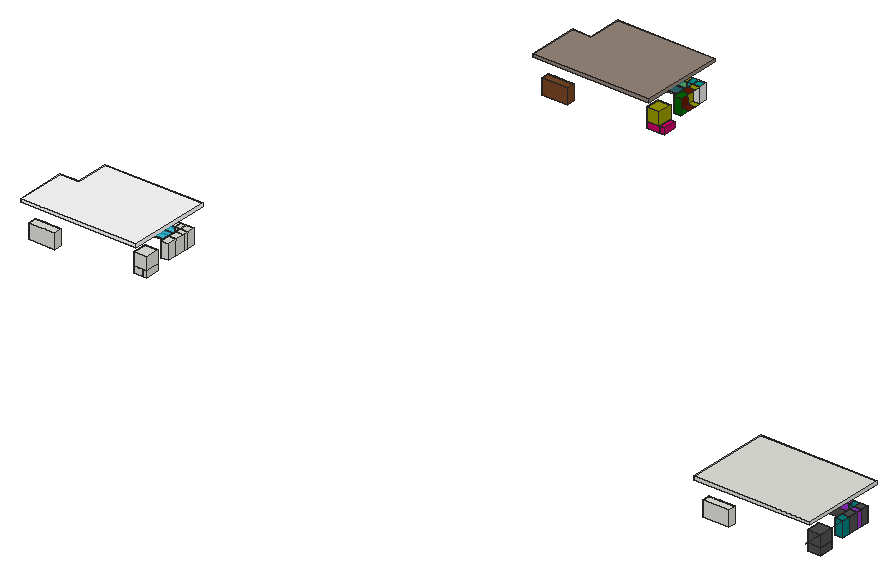
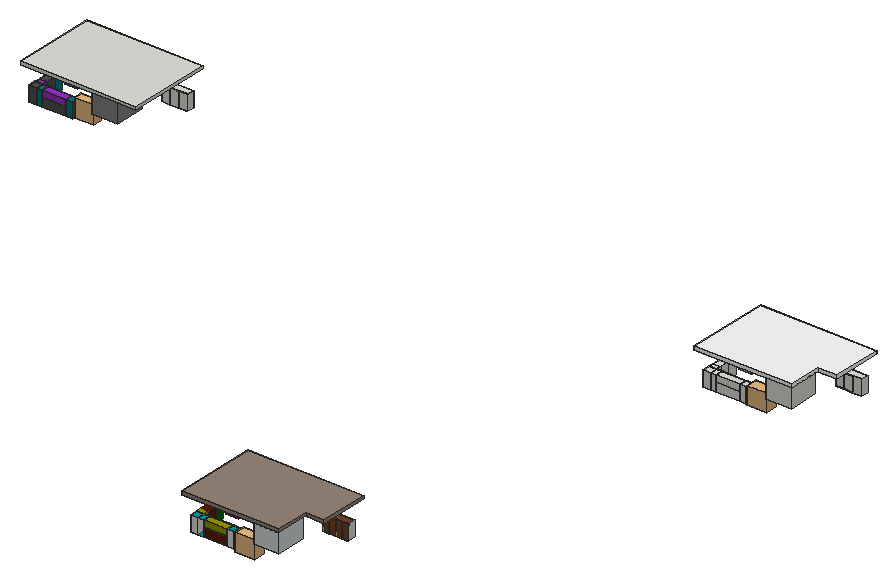
# SketchUp Ruby script. Lengths in inches.
U = 1.inch
M = Sketchup.active_model
def pt(a) = Geom::Point3d.new(a.map { |v| v * U })
def face(e, loops, mat)
  f = e.add_face(loops[0].map { |a| pt(a) })
  loops[1..].each { |l| e.add_face(l.map { |a| pt(a) }).erase! }
  f.material = f.back_material = mat if mat
  f
end
# faces: each face lists its corners as indices into pts; further lists are holes
def faces(e, pts, list, mat = nil) = list.each { |f| face(e, (f[0].is_a?(Array) ? f : [f]).map { |l| l.map { |i| pts[i] } }, mat) }
# xy, xz, yz: faces in a plane at the given z, y or x. An outline is a flat list of corners, or four numbers for a rectangle; further outlines are holes
def ring(l) = l.size == 4 ? [[l[0], l[1]], [l[2], l[1]], [l[2], l[3]], [l[0], l[3]]] : l.each_slice(2).to_a
def flat(e, list, mat, &to3) = list.each { |f| face(e, (f[0].is_a?(Array) ? f : [f]).map { |l| ring(l).map { |u, v| to3.(u, v) } }, mat) }
def xy(e, z, list, mat = nil) = flat(e, list, mat) { |x, y| [x, y, z] }
def xz(e, y, list, mat = nil) = flat(e, list, mat) { |x, z| [x, y, z] }
def yz(e, x, list, mat = nil) = flat(e, list, mat) { |y, z| [x, y, z] }
def lines(e, pts, list) = list.each { |a, b| e.add_line(pt(pts[a]), pt(pts[b])) }
# prism: a flat outline (further loops are holes) pulled along v
def prism(e, loops, v, mat = nil)
  f = face(e, loops, mat); d = Geom::Vector3d.new(v.map { |x| x * U })
  f.pushpull(f.normal.samedirection?(d) ? d.length : -d.length)
end
def box(e, o, s, mat = nil) = prism(e, [[o, [o[0] + s[0], o[1], o[2]], [o[0] + s[0], o[1] + s[1], o[2]], [o[0], o[1] + s[1], o[2]]]], [0, 0, s[2]], mat)
def at(x, y, z, deg = 0) = Geom::Transformation.translation(pt([x, y, z])) * Geom::Transformation.rotation(ORIGIN, Z_AXIS, deg.degrees)
def axes(o, x, y, z) = Geom::Transformation.new([*x, 0, *y, 0, *z, 0, *pt(o).to_a, 1])
def part(name) = M.definitions.add(name)
# library, detail: a bought-in or finely detailed component or shape, given as its bounding box
def library(name, o, s) = part(name).tap { |d| box(d.entities, o, s) }
def detail(e, o, s) = box(e.add_group.entities, o, s)
def put(e, d, t, mat = nil) = e.add_instance(d, t).tap { |i| i.material = mat if mat }
def group(e, t, mat = nil) = e.add_group.tap { |g| g.transformation = t; g.material = mat if mat }.entities
root = M.entities
M.materials.add("Wood 005 27.48cm\#1").color = [255, 255, 255]
M.materials.add("[0003_DeepPink]").color = [255, 20, 147]
M.materials.add("[0079_Teal]").color = [0, 128, 128]
M.materials.add("[0122_DarkOrchid]").color = [153, 50, 204]
M.materials.add("[0135_DarkGray]").color = [81, 81, 81]
M.materials.add("[Aluminum]").color = [179, 179, 179]
M.materials.add("[Brick Tumbled]").color = [135, 132, 132]
M.materials.add("[Carpet Berber Multi]").color = [151, 134, 122]
M.materials.add("[Color B08]").color = [102, 25, 0]
M.materials.add("[Color E07]").color = [153, 153, 0]
M.materials.add("[Color G08]").color = [0, 102, 0]
M.materials.add("[Color H07]").color = [0, 153, 153]
M.materials.add("[Color L06]").color = [204, 0, 100]
M.materials.add("[Metal Steel Textured]").color = [106, 110, 123]
M.materials.add("[Translucent Glass Dark Green]").color = [62, 91, 5]
M.materials["[Translucent Glass Dark Green]"].alpha = 0.5
M.materials.add("[Translucent Glass Tinted]").color = [8, 201, 241]
M.materials["[Translucent Glass Tinted]"].alpha = 0.48
M.materials.add("[Wallpaper Dog Bone]").color = [213, 224, 224]
M.materials.add("[Wood Veneer 01]").color = [120, 70, 37]
c1 = library("1-MICRO H40 CLC2",[0,-1.46,0],[23.5,21.66,15.63])
c2 = library("1-HOTTE ASPIRANTE CLC2",[-18.13,-19.43,-0.03],[36.22,19.49,31.49])
c3 = library("4-POIGNEE CLC2",[-3.31,-0.47,0],[6.61,0.94,1.5])
c4 = library("3-HOTTE ASPIRANTE CLC2",[-17.72,-15.75,0],[35.44,15.75,33])
c5 = part("Group\#8")
prism(c5.entities,[[[0,0,0],[0,90.79,0],[33.46,90.79,0],[33.46,151.42,0],[210.87,151.42,0],[210.87,0,0]]],[0,0,5.91])
xy(root,56.69,[[494.57,977.84,508.35,994.57],[441.42,1003.71,484.73,1004.42],[441.42,1004.42,484.73,1018.2]],"[Color B08]")
xy(root,56.69,[[494.57,994.57,508.35,1004.42]],"[Color E07]")
xy(root,56.69,[[494.57,961.11,508.35,977.84]],"[Color G08]")
xy(root,56.69,[[429.61,1004.42,441.42,1018.2],[484.73,1004.42,494.57,1018.2],[494.57,1004.42,508.35,1018.2]],"[Color H07]")
xy(root,56.69,[[315.4375,884.73,362.68,898.51]],"[Wood Veneer 01]")
xy(root,56.75,[[315.5,898.51,327.1875,899.22],[327.31,898.51,339,899.22],[339.12,898.51,350.8125,899.22],[350.93,898.51,362.62,899.22]],"[Wood Veneer 01]")
xy(root,56.8125,[[429.73,1003.71,441.3,1004.42]],"[Color H07]")
xy(root,57.4,[[442.13,1003.71,484.02,1003.86]],"[Aluminum]")
xy(root,57.4,[[442.13,1003.86,484.02,1004.42],[442.13,1004.42,484.02,1017.49]],"[Color B08]")
xy(root,71.73,[[442.13,1003.71,484.02,1003.86],[442.13,1003.86,484.02,1004.42],[442.13,1004.42,484.02,1017.49]],"[Color B08]")
xy(root,72.44,[[441.42,1003.71,484.73,1004.42]],"[Color E07]")
xy(root,73.15,[[442.13,1003.71,484.02,1004.0625]],"[Aluminum]")
xy(root,73.15,[[442.13,1004.0625,484.02,1004.42],[442.13,1004.42,484.02,1017.49]],"[Color E07]")
xy(root,83.54,[[442.13,1003.71,484.02,1004.0625]],"[Aluminum]")
xy(root,83.54,[[442.13,1004.0625,484.02,1004.42],[442.13,1004.42,484.02,1017.49]],"[Color E07]")
xy(root,84.13,[[429.73,1003.71,441.3,1004.42]],"[Color H07]")
xy(root,84.19,[[315.5,898.51,327.1875,899.22],[327.31,898.51,339,899.22],[339.12,898.51,350.8125,899.22],[350.93,898.51,362.62,899.22]],"[Wood Veneer 01]")
xy(root,84.25,[[441.42,1003.71,484.73,1004.42]],"[Aluminum]")
xy(root,84.25,[[494.57,977.84,508.35,994.57]],"[Color B08]")
xy(root,84.25,[[494.57,994.57,508.35,1004.42],[441.42,1004.42,484.73,1018.2]],"[Color E07]")
xy(root,84.25,[[494.57,961.11,508.35,977.84]],"[Color G08]")
xy(root,84.25,[[429.61,1004.42,441.42,1018.2],[484.73,1004.42,494.57,1018.2],[494.57,1004.42,508.35,1018.2]],"[Color H07]")
xy(root,84.25,[[315.4375,884.73,362.68,898.51]],"[Wood Veneer 01]")
xz(root,884.73,[[315.4375,56.69,362.68,84.25]],"[Wood Veneer 01]")
xz(root,898.51,[[[315.4375,56.69,327.25,84.25],[315.5,56.75,327.1875,84.19]],[[327.25,56.69,339.06,84.25],[327.31,56.75,339,84.19]],[[339.06,56.69,350.87,84.25],[339.12,56.75,350.8125,84.19]],[[350.87,56.69,362.68,84.25],[350.93,56.75,362.62,84.19]]],"[Wood Veneer 01]")
xz(root,899.22,[[315.5,56.75,327.1875,84.19],[327.31,56.75,339,84.19],[339.12,56.75,350.8125,84.19],[350.93,56.75,362.62,84.19]],"[Wood Veneer 01]")
xz(root,961.11,[[494.57,56.69,508.35,84.25]],"[Color G08]")
xz(root,1003.71,[[[441.42,56.69,484.73,72.44],[442.13,57.4,484.02,71.73]],[[441.42,72.44,484.73,84.25],[442.13,73.15,484.02,83.54]]],"[Aluminum]")
xz(root,1003.71,[[429.73,56.8125,441.3,84.13]],"[Color H07]")
xz(root,1003.86,[[442.13,57.4,484.02,71.73]],"[Translucent Glass Tinted]")
xz(root,1004.0625,[[442.13,73.15,484.02,83.54]],"[Translucent Glass Tinted]")
xz(root,1004.42,[[494.57,56.69,508.35,84.25]])
xz(root,1004.42,[[[441.42,56.69,484.73,72.44],[442.13,57.4,484.02,71.73]]],"[Color B08]")
xz(root,1004.42,[[[441.42,72.44,484.73,84.25],[442.13,73.15,484.02,83.54]]],"[Color E07]")
xz(root,1004.42,[[[429.61,56.69,441.42,84.25],[429.73,56.8125,441.3,84.13]],[484.73,56.69,494.57,84.25]],"[Color H07]")
xz(root,1017.49,[[442.13,57.4,484.02,71.73]],"[Color B08]")
xz(root,1017.49,[[442.13,73.15,484.02,83.54]],"[Color E07]")
xz(root,1018.2,[[429.61,56.69,441.42,84.25],[494.57,56.69,508.35,84.25]])
yz(root,315.4375,[[884.73,56.69,898.51,84.25]])
yz(root,315.5,[[898.51,56.75,899.22,84.19]],"[Wood Veneer 01]")
yz(root,327.1875,[[898.51,56.75,899.22,84.19]],"[Wood Veneer 01]")
yz(root,327.31,[[898.51,56.75,899.22,84.19]],"[Wood Veneer 01]")
yz(root,339,[[898.51,56.75,899.22,84.19]],"[Wood Veneer 01]")
yz(root,339.12,[[898.51,56.75,899.22,84.19]],"[Wood Veneer 01]")
yz(root,350.8125,[[898.51,56.75,899.22,84.19]],"[Wood Veneer 01]")
yz(root,350.93,[[898.51,56.75,899.22,84.19]],"[Wood Veneer 01]")
yz(root,362.62,[[898.51,56.75,899.22,84.19]],"[Wood Veneer 01]")
yz(root,362.68,[[884.73,56.69,898.51,84.25]],"[Wood Veneer 01]")
yz(root,429.61,[[1004.42,56.69,1018.2,84.25]],"[Color H07]")
yz(root,429.73,[[1003.71,56.8125,1004.42,84.13]],"[Color H07]")
yz(root,441.3,[[1003.71,56.8125,1004.42,72.44],[1003.71,72.44,1004.42,84.13]],"[Color H07]")
yz(root,441.42,[[1004.42,56.69,1018.2,72.44],[1004.42,72.44,1018.2,84.25]])
yz(root,441.42,[[1003.71,56.69,1004.42,72.44],[1003.71,72.44,1004.42,84.25]],"[Aluminum]")
yz(root,442.13,[[1003.71,57.4,1003.86,71.73],[1003.71,73.15,1004.0625,83.54]],"[Aluminum]")
yz(root,442.13,[[1003.86,57.4,1004.42,71.73],[1004.42,57.4,1017.49,71.73]],"[Color B08]")
yz(root,442.13,[[1004.0625,73.15,1004.42,83.54],[1004.42,73.15,1017.49,83.54]],"[Color E07]")
yz(root,484.02,[[1003.71,57.4,1003.86,71.73],[1003.71,73.15,1004.0625,83.54]],"[Aluminum]")
yz(root,484.02,[[1003.86,57.4,1004.42,71.73],[1004.42,57.4,1017.49,71.73]],"[Color B08]")
yz(root,484.02,[[1004.0625,73.15,1004.42,83.54],[1004.42,73.15,1017.49,83.54]],"[Color E07]")
yz(root,484.73,[[1003.71,56.69,1004.42,72.44],[1003.71,72.44,1004.42,84.25]],"[Aluminum]")
yz(root,494.57,[[1004.42,56.69,1018.2,84.25]])
yz(root,494.57,[[977.84,56.69,994.57,84.25]],"[Color B08]")
yz(root,494.57,[[994.57,56.69,1004.42,84.25]],"[Color E07]")
yz(root,494.57,[[961.11,56.69,977.84,84.25]],"[Color G08]")
yz(root,508.35,[[1004.42,56.69,1018.2,84.25]])
p = [[1380.78,196.16,62.69],[1380.78,196.16,90.25],[1459.52,196.16,90.25],[1445.74,196.16,90.25],[1392.59,196.16,62.69],[1392.59,196.16,78.44],
  [1459.52,196.16,62.69],[1445.74,196.16,62.69],[1435.9,196.16,90.25],[1435.9,196.16,78.44],[1459.52,155.81,90.25],[1459.52,155.81,62.69],
  [1459.52,138.37,90.25],[1459.52,114.75,90.25],[1459.52,89.16,90.25],[1459.52,182.38,62.69],[1459.52,182.38,90.25],[1392.59,196.16,90.25],
  [1435.9,196.16,62.69],[1459.52,114.75,67.97],[1459.52,89.16,67.97],[1459.52,114.75,55.84],[1459.52,89.16,55.84],[1459.52,139.08,90.25],
  [1459.52,139.08,62.69],[1459.52,172.54,90.25],[1459.52,138.37,62.69],[1459.52,71.4375,90.25],[1459.52,172.54,62.69],[1266.61,62.7,90.25],
  [1266.61,76.48,90.25],[1459.52,53.72,90.25],[1266.61,62.7,62.69],[1266.61,76.48,62.69]]
lines(root,p,[[0,1],[2,3],[4,5],[6,7],[8,9],[10,11],[12,13],[13,14],[15,16],[8,17],[7,3],[5,17],
  [7,18],[4,0],[9,18],[17,1],[18,4],[9,5],[19,20],[3,8],[21,22],[6,15],[2,16],[23,24],
  [25,10],[20,14],[24,26],[14,27],[25,28],[29,30],[21,19],[27,31],[23,12],[19,13],[22,20],[10,23],
  [32,29],[11,24],[6,2],[28,11],[15,28],[16,25],[26,12],[30,33]])
g1 = group(root,at(201.89,153.54,49.84))
xy(g1,0,[[-23.54,-25.59,-22.83,0],[-22.83,-25.59,0,0]])
xy(g1,0.35,[[-23.54,-24.88,-23.39,-0.71],[-23.39,-24.88,-23.1875,-0.71],[-23.1875,-24.88,-22.83,-0.71],[-22.83,-24.88,-8.07,-0.71]])
xy(g1,11.42,[[-23.54,-24.88,-23.39,-0.71],[-23.39,-24.88,-23.1875,-0.71],[-23.1875,-24.88,-22.83,-0.71],[-22.83,-24.88,-8.07,-0.71]])
xy(g1,12.125,[[-23.54,-25.59,-22.83,0],[-22.83,-25.59,0,0]])
xz(g1,-25.59,[[-23.54,0,-22.83,12.125],[-22.83,0,0,12.125]])
xz(g1,-24.88,[[-23.54,0.35,-23.39,11.42],[-23.39,0.35,-23.1875,11.42],[-23.1875,0.35,-22.83,11.42],[-22.83,0.35,-8.07,11.42]])
xz(g1,-0.71,[[-23.54,0.35,-23.39,11.42],[-23.39,0.35,-23.1875,11.42],[-23.1875,0.35,-22.83,11.42],[-22.83,0.35,-8.07,11.42]])
xz(g1,0,[[-23.54,0,-22.83,12.125],[-22.83,0,0,12.125]])
yz(g1,-23.54,[[[-25.59,0,0,12.125],[-24.88,0.35,-0.71,11.42]]])
yz(g1,-23.39,[[-24.88,0.35,-0.71,11.42]],"[Translucent Glass Dark Green]")
yz(g1,-23.1875,[[-24.88,0.35,-0.71,11.42]],"[Translucent Glass Dark Green]")
yz(g1,-22.83,[[[-25.59,0,0,12.125],[-24.88,0.35,-0.71,11.42]]])
yz(g1,-8.07,[[-24.88,0.35,-0.71,11.42]])
yz(g1,0,[[-25.59,0,0,12.125]])
g2 = group(root,at(508.35,936.78,49.84),"[Color L06]")
xy(g2,0,[[-22.83,-25.59,0,0]])
xy(g2,0.71,[[-22.83,-24.88,8.98,-0.71]])
xy(g2,11.42,[[-22.83,-24.88,8.98,-0.71]])
xy(g2,12.125,[[-22.83,-25.59,0,0]])
xz(g2,-25.59,[[-22.83,0,0,12.125]])
xz(g2,-24.88,[[-22.83,0.71,8.98,11.42]])
xz(g2,-0.71,[[-22.83,0.71,8.98,11.42]])
xz(g2,0,[[-22.83,0,0,12.125]])
yz(g2,-22.83,[[[-25.59,0,0,12.125],[-24.88,0.71,-0.71,11.42]]])
yz(g2,8.98,[[-24.88,0.71,-0.71,11.42]])
put(root,c1,axes([487.05,936.12,49.96],[0,-1.02666,0],[1.05455,0,0],[0,0,0.72267]))
put(root,c2,at(408.71,1018.2,52.68))
g3 = group(root,at(1459.52,114.75,55.84),"[0135_DarkGray]")
xy(g3,0,[[-22.83,-25.59,0,0]])
xy(g3,0.35,[[-22.83,-24.88,-0.71,-0.71]])
xy(g3,11.42,[[-22.83,-24.88,-0.71,-0.71]])
xy(g3,12.125,[[-22.83,-25.59,0,0]])
xz(g3,-25.59,[[-22.83,0,0,12.125]])
xz(g3,-24.88,[[-22.83,0.35,-0.71,11.42]])
xz(g3,-0.71,[[-22.83,0.35,-0.71,11.42]])
xz(g3,0,[[-22.83,0,0,12.125]])
yz(g3,-22.83,[[[-25.59,0,0,12.125],[-24.88,0.35,-0.71,11.42]]])
yz(g3,-0.71,[[-24.88,0.35,-0.71,11.42]])
yz(g3,0,[[-25.59,0,0,12.125]])
put(root,c2,at(103.08,234.95,55.9))
g4 = group(root,at(178.27,234.95,56.69))
xy(g4,0,[[0,-13.78,9.84,0]])
xy(g4,0.12,[[0.12,-14.49,8.21,-13.78]])
xy(g4,27.44,[[0.12,-14.49,8.21,-13.78]])
xy(g4,27.56,[[0,-13.78,9.84,0]])
xz(g4,-14.49,[[0.12,0.12,8.21,27.44]])
xz(g4,-13.78,[[[0,0,9.84,27.56],[0.12,0.12,9.72,27.44]],[8.21,0.12,8.27,27.44],[8.27,0.12,9.72,27.44]])
xz(g4,0,[[0,0,9.84,27.56]])
yz(g4,0,[[-13.78,0,0,15.75],[-13.78,15.75,0,27.56]])
yz(g4,0.12,[[-14.49,0.12,-13.78,15.75],[-14.49,15.75,-13.78,27.44]])
yz(g4,8.21,[[-14.49,0.12,-13.78,27.44]])
yz(g4,9.84,[[-13.78,0,0,27.56]])
g5 = group(root,at(134.96,234.95,56.69))
xy(g5,0,[[0,-14.49,43.31,-13.78],[0,-13.78,43.31,0]])
xy(g5,0.12,[[0.12,-14.33,43.1875,-14.13],[0.12,-14.13,43.1875,-13.78],[0.12,-13.78,43.1875,-0.47]])
xy(g5,0.12,[[0.12,-14.49,43.1875,-14.33]],"[Metal Steel Textured]")
xy(g5,15.63,[[0.12,-14.33,43.1875,-14.13],[0.12,-14.13,43.1875,-13.78],[0.12,-13.78,43.1875,-0.47]])
xy(g5,15.63,[[0.12,-14.49,43.1875,-14.33]],"[Metal Steel Textured]")
xy(g5,15.75,[[0,-14.49,43.31,-13.78],[0,-13.78,43.31,0]])
xz(g5,-14.49,[[[0,0,43.31,15.75],[0.12,0.12,43.1875,15.63]]],"[Metal Steel Textured]")
xz(g5,-14.33,[[0.12,0.12,43.1875,15.63]],"[Translucent Glass Tinted]")
xz(g5,-14.13,[[0.12,0.12,43.1875,15.63]],"[Translucent Glass Tinted]")
xz(g5,-13.78,[[[0,0,43.31,15.75],[0.12,0.12,43.1875,15.63]]])
xz(g5,-0.47,[[0.12,0.12,43.1875,15.63]])
xz(g5,0,[[0,0,43.31,15.75]])
yz(g5,0,[[-14.49,0,-13.78,15.75],[-13.78,0,0,15.75]])
yz(g5,0.12,[[-14.33,0.12,-14.13,15.63],[-14.13,0.12,-13.78,15.63],[-13.78,0.12,-0.47,15.63]])
yz(g5,0.12,[[-14.49,0.12,-14.33,15.63]],"[Metal Steel Textured]")
yz(g5,43.1875,[[-14.33,0.12,-14.13,15.63],[-14.13,0.12,-13.78,15.63],[-13.78,0.12,-0.47,15.63]])
yz(g5,43.1875,[[-14.49,0.12,-14.33,15.63]],"[Metal Steel Textured]")
yz(g5,43.31,[[-14.49,0,-13.78,15.75],[-13.78,0,0,15.75]])
g6 = group(root,at(123.15,234.95,56.69))
xy(g6,0,[[0,-13.78,11.8125,0]])
xy(g6,0.12,[[0.12,-14.49,11.69,-13.78]])
xy(g6,27.44,[[0.12,-14.49,11.69,-13.78]])
xy(g6,27.56,[[0,-13.78,11.8125,0]])
xz(g6,-14.49,[[0.12,0.12,11.69,27.44]])
xz(g6,-13.78,[[[0,0,11.8125,27.56],[0.12,0.12,11.69,27.44]]])
xz(g6,0,[[0,0,11.8125,27.56]])
yz(g6,0,[[-13.78,0,0,27.56]])
yz(g6,0.12,[[-14.49,0.12,-13.78,27.44]])
yz(g6,11.69,[[-14.49,0.12,-13.78,15.75],[-14.49,15.75,-13.78,27.44]])
yz(g6,11.8125,[[-13.78,0,0,15.75],[-13.78,15.75,0,27.56]])
g7 = group(root,at(8.98,115.27,56.69))
xy(g7,0,[[0,-13.78,47.24,0]])
xy(g7,27.56,[[0,-13.78,47.24,0]])
xz(g7,-13.78,[[0,0,47.24,27.56]])
xz(g7,0,[[[0,0,15.75,27.56],[0.12,0.12,15.63,27.44]],[[15.75,0,31.5,27.56],[15.87,0.12,31.38,27.44]],[[31.5,0,47.24,27.56],[31.61,0.12,47.125,27.44]],[0.12,0.12,15.63,27.44],[15.87,0.12,31.38,27.44],
  [31.61,0.12,47.125,27.44]])
yz(g7,0,[[-13.78,0,0,27.56]])
yz(g7,47.24,[[-13.78,0,0,27.56]])
g8 = group(root,at(201.89,194.6,56.69))
xy(g8,0,[[-13.78,-16.73,0,0]])
xy(g8,0.06,[[-14.49,-16.67,-13.78,-0.06]])
xy(g8,27.5,[[-14.49,-16.67,-13.78,-0.06]])
xy(g8,27.56,[[-13.78,-16.73,0,0]])
xz(g8,-16.73,[[-13.78,0,0,27.56]])
xz(g8,-16.67,[[-14.49,0.06,-13.78,27.5]])
xz(g8,-0.06,[[-14.49,0.06,-13.78,27.5]])
xz(g8,0,[[-13.78,0,0,27.56]])
yz(g8,-14.49,[[-16.67,0.06,-0.06,27.5]])
yz(g8,-13.78,[[[-16.73,0,0,27.56],[-16.67,0.06,-0.06,27.5]]])
yz(g8,0,[[-16.73,0,0,27.56]])
g9 = group(root,at(201.89,211.33,56.69))
xy(g9,0,[[-13.78,-16.73,0,0]])
xy(g9,0.06,[[-14.49,-16.67,-13.78,-0.06]])
xy(g9,27.5,[[-14.49,-16.67,-13.78,-0.06]])
xy(g9,27.56,[[-13.78,-16.73,0,0]])
xz(g9,-16.73,[[-13.78,0,0,27.56]])
xz(g9,-16.67,[[-14.49,0.06,-13.78,27.5]])
xz(g9,-0.06,[[-14.49,0.06,-13.78,27.5]])
xz(g9,0,[[-13.78,0,0,27.56]])
yz(g9,-14.49,[[-16.67,0.06,-0.06,27.5]])
yz(g9,-13.78,[[[-16.73,0,0,27.56],[-16.67,0.06,-0.06,27.5]]])
yz(g9,0,[[-16.73,0,0,27.56]])
g10 = group(root,at(201.89,234.95,56.69))
box(g10,[-13.78,-13.78,0],[13.78,13.78,27.56])
g11 = group(root,at(201.89,221.17,56.69))
xy(g11,0,[[-13.78,-9.84,0,0]])
xy(g11,0.12,[[-14.49,-9.72,-13.78,-1.69]])
xy(g11,27.44,[[-14.49,-9.72,-13.78,-1.69]])
xy(g11,27.56,[[-13.78,-9.84,0,0]])
xz(g11,-9.84,[[-13.78,0,0,27.56]])
xz(g11,-9.72,[[-14.49,0.12,-13.78,27.44]])
xz(g11,-1.69,[[-14.49,0.12,-13.78,27.44]])
xz(g11,0,[[-13.78,0,0,27.56]])
yz(g11,-14.49,[[-9.72,0.12,-1.69,27.44]])
yz(g11,-13.78,[[[-9.84,0,0,27.56],[-9.72,0.12,-0.12,27.44]],[-1.69,0.12,-1.57,27.44],[-1.57,0.12,-0.12,27.44]])
yz(g11,0,[[-9.84,0,0,27.56]])
put(root,c3,axes([337.53,899.22,61.17],[0,0,1],[1,0,0],[0,1,0]))
put(root,c3,axes([349.34,899.22,61.17],[0,0,1],[1,0,0],[0,1,0]))
put(root,c3,axes([325.72,899.22,61.17],[0,0,1],[1,0,0],[0,1,0]))
put(root,c3,axes([361.15,899.22,61.17],[0,0,1],[1,0,0],[0,1,0]))
g12 = group(root,at(201.89,153.54,61.97))
xy(g12,0,[[-22.83,-25.59,0,0]])
xy(g12,0.06,[[-23.54,-25.53,-22.83,-0.06]])
xy(g12,22.22,[[-23.54,-25.53,-22.83,-0.06]])
xy(g12,22.28,[[-22.83,-25.59,0,0]])
xz(g12,-25.59,[[-22.83,0,0,22.28]])
xz(g12,-25.53,[[-23.54,0.06,-22.83,22.22]])
xz(g12,-0.06,[[-23.54,0.06,-22.83,22.22]])
xz(g12,0,[[-22.83,0,0,22.28]])
yz(g12,-23.54,[[-25.53,0.06,-0.06,22.22]])
yz(g12,-22.83,[[[-25.59,0,0,22.28],[-25.53,0.06,-0.06,22.22]]])
yz(g12,0,[[-25.59,0,0,22.28]])
g13 = group(root,at(508.35,936.78,61.97),"[Color E07]")
xy(g13,0,[[-22.83,-25.59,0,0]])
xy(g13,22.28,[[-22.83,-25.59,0,0]])
xz(g13,-25.59,[[-22.83,0,0,22.28]])
xz(g13,0,[[-22.83,0,0,22.28]])
yz(g13,-22.83,[[[-25.59,0,0,22.28],[-25.53,0.06,-0.06,22.22]],[-25.53,0.06,-0.06,22.22]])
yz(g13,0,[[-25.59,0,0,22.28]])
g14 = group(root,at(1266.61,62.7,62.69))
xy(g14,0,[[0,0,47.24,13.78]])
xy(g14,27.56,[[0,0,47.24,13.78]])
xz(g14,0,[[0,0,47.24,27.56]])
xz(g14,13.78,[[[0,0,15.75,27.56],[0.12,0.12,15.63,27.44]],[[15.75,0,31.5,27.56],[15.87,0.12,31.38,27.44]],[[31.5,0,47.24,27.56],[31.61,0.12,47.125,27.44]]])
yz(g14,0,[[0,0,13.78,27.56]])
yz(g14,47.24,[[0,0,13.78,27.56]])
g15 = group(root,at(1459.52,155.81,62.69),"[0079_Teal]")
box(g15,[-13.78,-16.73,0],[13.78,16.73,27.56])
g16 = group(root,at(1459.52,172.54,62.69),"[0135_DarkGray]")
box(g16,[-13.78,-16.73,0],[13.78,16.73,27.56])
g17 = group(root,at(1459.52,196.16,62.69),"[0003_DeepPink]")
box(g17,[-13.78,-13.78,0],[13.78,13.78,27.56])
g18 = group(root,at(1459.52,182.38,62.69),"[0122_DarkOrchid]")
box(g18,[-13.78,-9.84,0],[13.78,9.84,27.56])
g19 = group(root,at(1445.74,196.16,62.69),"[0135_DarkGray]")
box(g19,[0,-13.78,0],[13.78,13.78,27.56])
g20 = group(root,at(1392.59,196.16,62.69),"[0135_DarkGray]")
box(g20,[0,-13.78,0],[43.31,13.78,15.75])
g21 = group(root,at(1435.9,196.16,62.69),"[0079_Teal]")
box(g21,[0,-13.78,0],[9.84,13.78,27.56])
g22 = group(root,at(1380.78,196.16,62.69),"[0079_Teal]")
box(g22,[0,-13.78,0],[11.8125,13.78,27.56])
g23 = group(root,at(1266.73,76.48,62.8125))
box(g23,[0,0,0],[15.51,0.71,27.32])
g24 = group(root,at(1282.47,76.48,62.8125))
box(g24,[0,0,0],[15.51,0.71,27.32])
g25 = group(root,at(1298.22,76.48,62.8125))
box(g25,[0,0,0],[15.51,0.71,27.32])
put(root,c4,at(1359.57,196.16,65.8))
g26 = group(root,at(1459.52,114.75,67.97),"[0135_DarkGray]")
xy(g26,0,[[-22.83,-25.59,0,0]])
xy(g26,0.06,[[-23.54,-25.53,-22.83,-0.06]])
xy(g26,22.22,[[-23.54,-25.53,-22.83,-0.06]])
xy(g26,22.28,[[-22.83,-25.59,0,0]])
xz(g26,-25.59,[[-22.83,0,0,22.28]])
xz(g26,-25.53,[[-23.54,0.06,-22.83,22.22]])
xz(g26,-0.06,[[-23.54,0.06,-22.83,22.22]])
xz(g26,0,[[-22.83,0,0,22.28]])
yz(g26,-23.54,[[-25.53,0.06,-0.06,22.22]])
yz(g26,-22.83,[[[-25.59,0,0,22.28],[-25.53,0.06,-0.06,22.22]]])
yz(g26,0,[[-25.59,0,0,22.28]])
g27 = group(root,at(134.96,234.95,72.44))
xy(g27,0,[[0,-14.49,43.31,-13.78],[0,-13.78,43.31,0]])
xy(g27,0.12,[[0.12,-14.33,43.1875,-14.13],[0.12,-13.78,43.1875,-0.47]])
xy(g27,0.12,[[0.12,-14.49,43.1875,-14.33],[0.12,-14.13,43.1875,-13.78]],"[Metal Steel Textured]")
xy(g27,11.69,[[0.12,-14.33,43.1875,-14.13],[0.12,-13.78,43.1875,-0.47]])
xy(g27,11.69,[[0.12,-14.49,43.1875,-14.33],[0.12,-14.13,43.1875,-13.78]],"[Metal Steel Textured]")
xy(g27,11.8125,[[0,-13.78,43.31,0]])
xy(g27,11.8125,[[0,-14.49,43.31,-13.78]],"[Metal Steel Textured]")
xz(g27,-14.49,[[[0,0,43.31,11.8125],[0.12,0.12,43.1875,11.69]]],"[Metal Steel Textured]")
xz(g27,-14.33,[[0.12,0.12,43.1875,11.69]],"[Translucent Glass Tinted]")
xz(g27,-14.13,[[0.12,0.12,43.1875,11.69]],"[Translucent Glass Tinted]")
xz(g27,-13.78,[[[0,0,43.31,11.8125],[0.12,0.12,43.1875,11.69]]])
xz(g27,-0.47,[[0.12,0.12,43.1875,11.69]])
xz(g27,0,[[0,0,43.31,11.8125]])
yz(g27,0,[[-13.78,0,0,11.8125]])
yz(g27,0,[[-14.49,0,-13.78,11.8125]],"[Metal Steel Textured]")
yz(g27,0.12,[[-14.33,0.12,-14.13,11.69],[-13.78,0.12,-0.47,11.69]])
yz(g27,0.12,[[-14.49,0.12,-14.33,11.69],[-14.13,0.12,-13.78,11.69]],"[Metal Steel Textured]")
yz(g27,43.1875,[[-14.33,0.12,-14.13,11.69],[-13.78,0.12,-0.47,11.69]])
yz(g27,43.1875,[[-14.49,0.12,-14.33,11.69],[-14.13,0.12,-13.78,11.69]],"[Metal Steel Textured]")
yz(g27,43.31,[[-14.49,0,-13.78,11.8125],[-13.78,0,0,11.8125]])
g28 = group(root,at(1392.59,196.16,78.44),"[0122_DarkOrchid]")
box(g28,[0,-13.78,0],[43.31,13.78,11.8125])
g29 = group(root,at(339.92,973.3125,84),"[Wallpaper Dog Bone]")
prism(g29,[[[0,53.86,0],[46.38,53.86,0],[46.38,44.88,0],[8.98,44.88,0],[8.98,0,0],[0,0,0]]],[0,0,34.11])
g30 = group(root,at(33.46,190.07,84.08))
prism(g30,[[[46.38,53.86,0],[46.38,44.88,0],[8.98,44.88,0],[8.98,0,0],[0,0,0],[0,53.86,0]]],[0,0,34.03])
g31 = group(root,at(1291.1,151.28,90),"[Brick Tumbled]")
prism(g31,[[[46.38,53.86,0],[46.38,44.88,0],[8.98,44.88,0],[8.98,0,0],[0,0,0],[0,53.86,0]]],[0,0,34.11])
g32 = group(root,at(0,92.51,118.11),"Wood 005 27.48cm\#1")
xy(g32,0,[[0,0,0,90.79,33.46,90.79,33.46,151.42,210.87,151.42,210.87,0]])
xy(g32,6,[[0,0,210.87,0,210.87,151.42,33.46,151.42,33.46,90.79,0,90.79]],"Wood 005 27.48cm\#1")
xz(g32,0,[[0,0,210.87,6]])
xz(g32,90.79,[[0,0,33.46,6]])
xz(g32,151.42,[[33.46,0,210.87,6]])
yz(g32,0,[[0,0,90.79,6]])
yz(g32,33.46,[[90.79,0,151.42,6]])
yz(g32,210.87,[[0,0,151.42,6]])
put(root,c5,at(306.46,875.75,118.11),"[Carpet Berber Multi]")
g33 = group(root,at(1257.63,53.72,124.11))
box(g33,[0,0,0],[210.87,151.42,6])
